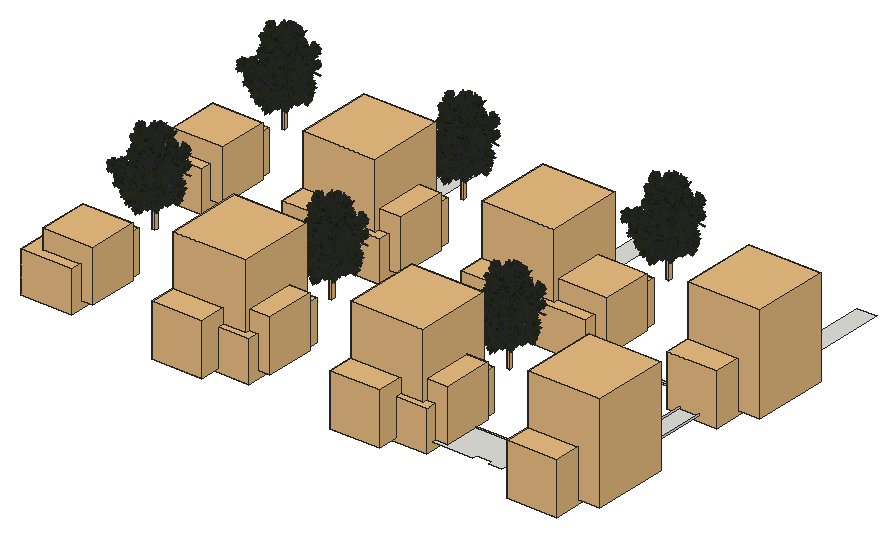
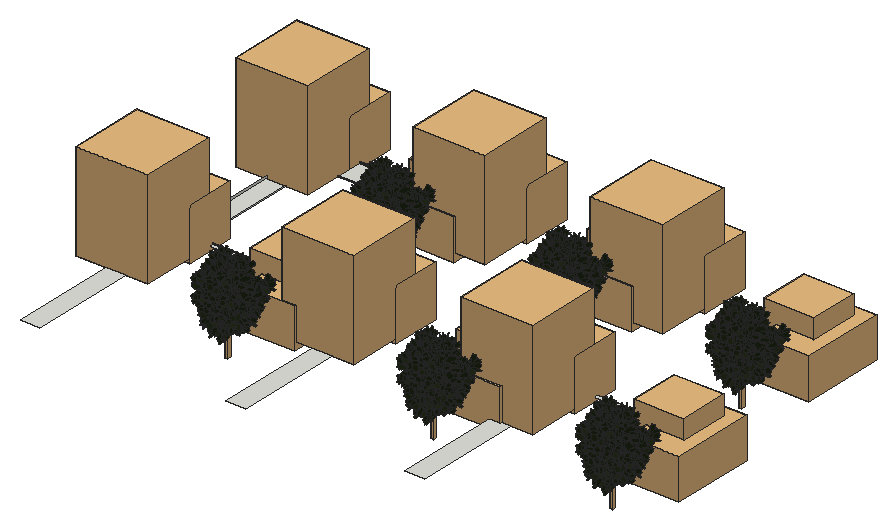
# SketchUp Ruby script. Lengths in inches.
U = 1.inch
M = Sketchup.active_model
def pt(a) = Geom::Point3d.new(a.map { |v| v * U })
def face(e, loops, mat)
  f = e.add_face(loops[0].map { |a| pt(a) })
  loops[1..].each { |l| e.add_face(l.map { |a| pt(a) }).erase! }
  f.material = f.back_material = mat if mat
  f
end
# faces: each face lists its corners as indices into pts; further lists are holes
def faces(e, pts, list, mat = nil) = list.each { |f| face(e, (f[0].is_a?(Array) ? f : [f]).map { |l| l.map { |i| pts[i] } }, mat) }
# xy, xz, yz: faces in a plane at the given z, y or x. An outline is a flat list of corners, or four numbers for a rectangle; further outlines are holes
def ring(l) = l.size == 4 ? [[l[0], l[1]], [l[2], l[1]], [l[2], l[3]], [l[0], l[3]]] : l.each_slice(2).to_a
def flat(e, list, mat, &to3) = list.each { |f| face(e, (f[0].is_a?(Array) ? f : [f]).map { |l| ring(l).map { |u, v| to3.(u, v) } }, mat) }
def xy(e, z, list, mat = nil) = flat(e, list, mat) { |x, y| [x, y, z] }
def xz(e, y, list, mat = nil) = flat(e, list, mat) { |x, z| [x, y, z] }
def yz(e, x, list, mat = nil) = flat(e, list, mat) { |y, z| [x, y, z] }
def lines(e, pts, list) = list.each { |a, b| e.add_line(pt(pts[a]), pt(pts[b])) }
# prism: a flat outline (further loops are holes) pulled along v
def prism(e, loops, v, mat = nil)
  f = face(e, loops, mat); d = Geom::Vector3d.new(v.map { |x| x * U })
  f.pushpull(f.normal.samedirection?(d) ? d.length : -d.length)
end
def box(e, o, s, mat = nil) = prism(e, [[o, [o[0] + s[0], o[1], o[2]], [o[0] + s[0], o[1] + s[1], o[2]], [o[0], o[1] + s[1], o[2]]]], [0, 0, s[2]], mat)
def at(x, y, z, deg = 0) = Geom::Transformation.translation(pt([x, y, z])) * Geom::Transformation.rotation(ORIGIN, Z_AXIS, deg.degrees)
def axes(o, x, y, z) = Geom::Transformation.new([*x, 0, *y, 0, *z, 0, *pt(o).to_a, 1])
def part(name) = M.definitions.add(name)
# library, detail: a bought-in or finely detailed component or shape, given as its bounding box
def library(name, o, s) = part(name).tap { |d| box(d.entities, o, s) }
def detail(e, o, s) = box(e.add_group.entities, o, s)
def put(e, d, t, mat = nil) = e.add_instance(d, t).tap { |i| i.material = mat if mat }
def group(e, t, mat = nil) = e.add_group.tap { |g| g.transformation = t; g.material = mat if mat }.entities
root = M.entities
M.materials.add("Green ash – green texture").color = [33, 41, 22]
M.materials.add("[Color_005]").color = [114, 114, 114]
M.materials.add("[Color_D09]").color = [86, 59, 49]
M.materials.add("[Pavers with Grass Herringbone]").color = [197, 201, 190]
c1 = part("Component\#13")
xz(c1.entities,0,[[2.54,0,9.87,0.64,10.99,2.07,11.4,3.42,15.13,2.28,14.48,4.31,16.14,5.21,16.14,6.08,19.81,7.28,19.6,9.67,17.45,11.49,17.45,12.16,18.82,14.37,17.48,14.37,14.41,13.66,14.41,15.23,12.5625,17.49,9.84,15.21,8.9,13.85,7.74,13.625,7.35,12.68,6.87,13.02,6.35,12.27,5.92,10.47,4.2,7.42,2.84,6.89,0,2.38,0.07,1.59,2.8125,4.94,3.37,3.59,2.54,3.37,2.12,2.22]],"Green ash – green texture")
c2 = part("Component\#14")
xz(c2.entities,0,[[1.1,0,1.61,0,2.73,1.11,4.34,2.72,5.21,6.36,5.85,7.16,6.35,6.9375,6.85,8.05,8.03,8.05,8.625,9.25,10.11,11.7,9.56,13.83,9.56,15.84,7.83,15.84,6.03,14.37,5.31,16.54,4.4375,17.39,1.45,14.31,0,9.15,1.4,5.18,3.01,6.08,1.98,1.39]],"Green ash – green texture")
c3 = part("Component\#16")
put(c3.entities,c1,axes([0,7.77,0],[1,0,0],[0,0.89571,0.44464],[0,-0.44464,0.89571]))
put(c3.entities,c2,axes([2.15,6.37,5.26],[0.57629,-0.80824,0.12095],[0.79263,0.51673,-0.3236],[0.19905,0.28236,0.93843]))
c4 = part("Component\#7")
put(c4.entities,c3,axes([-4.97,-3.22,4.05],[0.69883,-0.69034,0.18725],[0.53248,0.3273,-0.7806],[0.47759,0.64522,0.59632]))
c5 = part("Component\#8")
put(c5.entities,c4,axes([0,5.2,2.2],[1,0,0],[0,0.90259,0.43051],[0,-0.43051,0.90259]))
c6 = part("leaf group 2")
put(c6.entities,c5,axes([-11.99,4.41,-4.35],[2.22014,-0.82385,1.14017],[1.36501,1.77637,-1.37441],[-0.33979,1.75315,1.92841]))
c7 = part("Component\#10")
put(c7.entities,c6,axes([-5.27,11.65,1.68],[-0.48323,0.10636,-0.43072],[-0.11515,-0.64511,-0.03012],[-0.42845,0.05342,0.49388]))
c8 = part("Component\#9")
xz(c8.entities,0,[[0.64,0,0,0.1875,4.21,2.81,8.59,4.11,12.8,4.11,19.57,2.81,12.8,3.73,8.59,3.73,4.21,2.3125]],"[Color_D09]")
c9 = part("Leafy twig")
put(c9.entities,c7,axes([23.53,12.57,24.85],[0.06536,-0.90475,-0.42089],[0.61791,-0.2945,0.72901],[-0.78353,-0.30772,0.53981]))
put(c9.entities,c7,axes([22.7,12.25,24.83],[-0.47146,-0.89493,0.11311],[0.80135,-0.48549,-0.35888],[0.36776,-0.0521,0.90651]))
put(c9.entities,c7,axes([24.25,0.65,20.83],[0.8253,-0.50372,0.24924],[0.23848,0.71461,0.65749],[-0.51157,-0.48438,0.71194]))
put(c9.entities,c7,axes([23.54,-2.45,18.63],[0.04689,-0.92492,0.3511],[0.72122,-0.28285,-0.64421],[0.71641,0.2674,0.65188]))
put(c9.entities,c7,axes([22.39,16.15,27.04],[-0.5311,-0.82173,0.2419],[0.41574,0.01583,0.89559],[-0.77461,0.50499,0.40813]))
put(c9.entities,c8,axes([22.76,-5.09,13.48],[0,1.66539,0.44624],[-1.72414,0,0],[0,-0.44624,1.66539]))
c10 = part("Component\#12")
p = [[0,0,0.13],[0.41,0.77,0],[4.07,2.79,10.125],[3.73,2.15,10.23],[7.66,4.77,23.875],[7.4,4.27,23.96],
  [8.6875,5.26,35.99],[8.5,4.91,36.05],[8.32,4.9375,46.95],[8.21,4.74,46.98]]
faces(c10.entities,p,[[0,1,2,3],[3,2,4,5],[4,6,7,5],[6,8,9,7]],"[Color_005]")
c11 = part("Leafy twig \#1")
put(c11.entities,c10,axes([3.13,0.17,-0.45],[3.38032,6.88592,0.52481],[-5.85488,3.97559,0.303],[0,-1.35912,3.54524]))
put(c11.entities,c7,axes([0.37,31.375,148.94],[0.47772,0.64064,-1.51139],[2.85768,-0.62659,0.20284],[-0.43926,-3.3797,-0.3241]))
c12 = part("Leafy branch \#1")
put(c12.entities,c9,axes([28.11,72.66,46.26],[0.77413,-0.41274,-0.47998],[0.6311,0.56229,0.53435],[0.04934,-0.71657,0.69577]))
put(c12.entities,c9,axes([31.25,3.94,9.17],[0.73236,0.67893,0.05208],[-0.46223,0.55185,-0.69413],[-0.5,0.48428,0.71797]))
put(c12.entities,c9,axes([20.16,84.84,57.95],[0.96628,0.19619,0.16678],[-0.2575,0.73909,0.62245],[-0.00115,-0.6444,0.76469]))
put(c12.entities,c9,axes([30.13,29.18,11.93],[0.86603,0.2796,0.41452],[0,0.82904,-0.55919],[-0.5,0.48428,0.71797]))
put(c12.entities,c9,axes([47.67,28.63,-3.7],[0.1205,-0.71255,0.69119],[0.96646,0.24327,0.08231],[-0.2268,0.65809,0.71797]))
put(c12.entities,c9,axes([48.76,50.64,76.31],[-0.6716,0.46861,-0.57389],[0.01402,0.78248,0.62252],[0.74078,0.41004,-0.53209]))
put(c12.entities,c11,axes([42.34,0,10.34],[0.39368,0,0],[0,0.22544,-0.24092],[0,0.54032,0.50562]))
put(c12.entities,c9,axes([64.51,80.82,101.08],[-0.99604,0.06562,-0.06004],[-0.0106,0.58266,0.81265],[0.08831,0.81006,-0.57966]))
c13 = library("Component\#18",[-6.35,9.4375,-76.57],[12.56,13.68,315.77])
c14 = part("Leafy branch \#3")
put(c14.entities,c9,axes([-3.64,36.17,23.18],[0.95801,0.10249,0.26779],[-0.28581,0.41631,0.86313],[-0.02302,-0.90343,0.42812]))
put(c14.entities,c9,axes([13.16,55.79,39.92],[0.70711,-0.61725,0.34497],[0,0.48786,0.87292],[-0.70711,-0.61725,0.34497]))
put(c14.entities,c11,axes([18.8125,5.17,0.46],[0.25503,0,0],[0,0.20007,-0.0752],[0,0.16866,0.44872]))
put(c14.entities,c9,axes([23.62,-10.17,21.5],[-0.56253,0.81775,0.12181],[0.38738,0.13053,0.91263],[0.73041,0.56057,-0.39021]))
put(c14.entities,c9,axes([45.18,27.18,68.96],[-0.96593,-0.22593,0.12627],[0.12295,0.02876,0.992],[-0.22775,0.97372,0]))
c15 = part("Component\#19")
put(c15.entities,c11,axes([21.47,3.93,0.22],[0.25503,0,0],[0,0.21068,-0.03601],[0,0.08077,0.47252]))
put(c15.entities,c9,axes([-4.05,13.6875,55.34],[0.70711,0.70373,-0.069],[0,0.09758,0.99523],[0.70711,-0.70373,0.069]))
put(c15.entities,c9,axes([6.52,33.54,18.07],[0.92587,-0.37604,0.03687],[0,0.09758,0.99523],[-0.37784,-0.92145,0.09035]))
c16 = part("Leafy branch \#2")
put(c16.entities,c9,axes([26.17,74.02,40.56],[0.25882,-0.64004,0.72344],[0,0.74896,0.66262],[-0.96593,-0.1715,0.19384]))
put(c16.entities,c9,axes([6.38,24.03,55.81],[-0.04786,0.8645,-0.50035],[0.15558,0.50126,0.85119],[0.98666,-0.03711,-0.15849]))
put(c16.entities,c11,axes([17.68,0,1.01],[0.32282,0,0],[0,0.21407,-0.16545],[0,0.37107,0.48011]))
put(c16.entities,c9,axes([-9.1875,31.15,28.07],[0.82314,0.37626,-0.42529],[0,0.74896,0.66262],[0.56784,-0.54543,0.61649]))
put(c16.entities,c9,axes([0.54,-12.07,9.94],[0.19622,0.90478,-0.37799],[-0.67396,0.40444,0.61823],[0.71224,0.13344,0.68914]))
put(c16.entities,c9,axes([7.34,9.15,39.57],[0.05153,0.73872,-0.67204],[0.38679,0.60565,0.6954],[0.92072,-0.29578,-0.25452]))
put(c16.entities,c9,axes([36.2,51.23,15.73],[-0.18626,-0.35374,0.91661],[-0.31641,0.90483,0.2849],[-0.93016,-0.23696,-0.28046]))
c17 = part("Tree")
put(c17.entities,c12,axes([-22.29,52.36,216.76],[0.38964,-1.07313,-0.10036],[1.06809,0.37236,0.19631],[-0.13881,-0.14712,1.22884]))
put(c17.entities,c12,axes([59.83,6.78,230.57],[-1.28826,-0.23008,-0.3647],[0.05148,-1.22938,0.51215],[-0.34663,0.55136,1.25774]))
put(c17.entities,c13,axes([-2.16,-18.04,104.22],[1.30157,0,0],[0,1.30157,0],[0,0,1.36111]))
put(c17.entities,c12,axes([-55.8,4.2,115.32],[1.30157,0,0],[0,1.29536,0.19359],[0,-0.26855,1.38538]))
put(c17.entities,c12,axes([5.36,-52.22,156.04],[-0.23532,1.19719,-0.71362],[-1.32974,0,0.39335],[0.40758,0.6912,1.23603]))
put(c17.entities,c14,axes([-20.09,22.57,317.7],[0,-1.33697,0],[1.33697,0,0],[0,0,1.4573]))
put(c17.entities,c12,axes([44.2,-31.84,172.82],[-1.11894,0.85085,0],[-0.85085,-1.11894,0],[0,0,1.53221]))
put(c17.entities,c12,axes([-10.2,63.7,119.93],[0.28716,-1.46366,0],[1.41378,0.27737,0.38604],[-0.41292,-0.08101,1.5704]))
put(c17.entities,c12,axes([-29.03,-40.72,232.79],[0.5211,0.98898,-0.38718],[-1.02974,0.58664,0.11255],[0.35577,0.28216,1.19957]))
put(c17.entities,c12,axes([44.92,21.7,135.38],[-1.05627,-0.44294,0],[0.44294,-1.05627,0],[0,0,1.24847]))
put(c17.entities,c14,axes([-32.94,-0.59,304.82],[1.2814,-0.22825,0],[0.22825,1.2814,0],[0,0,1.41871]))
put(c17.entities,c14,axes([0.6,-31.29,315.98],[0.13082,1.33422,0],[-1.33422,0.13082,0],[0,0,1.46127]))
put(c17.entities,c14,axes([21.3,1.66,315.16],[-1.25722,0.32198,-0.09905],[-0.32539,-1.26867,0.00612],[-0.08719,0.09194,1.40547]))
put(c17.entities,c15,axes([-19,30.84,372.72],[0.65078,-1.12719,0],[1.12719,0.65078,0],[0,0,1.41871]))
put(c17.entities,c15,axes([14.39,-16.125,357],[-0.73695,1.06095,0.15933],[-1.03698,-0.75397,0.2242],[0.29981,0,1.38667]))
put(c17.entities,c16,axes([-5.9,-20.03,270.39],[0,1.47598,0],[-1.4157,0,0.41751],[0.45509,0,1.54311]))
put(c17.entities,c16,axes([-18.4375,22.18,263.88],[0.84243,-1.42226,-0.32685],[1.40385,0.7063,0.64743],[-0.37678,-0.54841,1.68147]))
put(c17.entities,c16,axes([-29.32,4.9,283.41],[1.35363,0,0],[0,1.33841,0.20242],[0,-0.22063,1.45887]))
put(c17.entities,c16,axes([17.31,11.65,257.52],[-1.14969,-0.5642,-0.25322],[0.46017,-1.12719,0.50159],[-0.40066,0.32434,1.3027]))
put(c17.entities,c16,axes([16.3,15.3125,240.45],[-0.98541,-0.85203,0.68095],[1.00747,-1.01506,0.22317],[0.31818,0.5753,1.40228]))
put(c17.entities,c12,axes([-46.75,22.93,206.12],[1.08363,-0.37101,0],[0.37101,1.08363,0],[0,0,1.24847]))
put(c17.entities,c12,axes([41.1,-35.18,99.125],[-1.05556,0.85173,0.25344],[-0.84493,-1.04965,0.12953],[0.39153,-0.09409,1.38106]))
c18 = library("VEGETAÇÃO+TROPICAL+EM+VASOS",[-14.15,-83.94,15.25],[179.21,109.09,86.78])
c19 = library("Plant+++Pot",[-21.48,-119.36,-205.6875],[86.44,86.43,89.41])
c20 = library("Plant",[0,0,0],[12.59,12.59,14.16])
c21 = library("ganyedes's+yellow&green+tree",[-30.91,-35.46,0],[63.51,67.02,85.79])
xy(root,-12.3125,[[2364.02,147.25,2435.71,305.58],[2140.42,162.33,2140.42,178.0625,2083.4,178.0625,2083.4,162.52,1785.21,162.52,1785.21,305.58,2364.02,305.58,2364.02,203.875,2347.875,203.875,2347.875,204.875,2347.125,204.875,2347.125,203.875,2343.875,203.875,2343.875,204.875,2343.125,204.875,2343.125,203.875,2339.875,203.875,2339.875,204.875,2339.125,204.875,2339.125,203.875,2335.875,203.875,2335.875,204.875,2335.125,204.875,2335.125,203.875,2331.875,203.875,2331.875,204.875,2331.125,204.875,2331.125,203.875,2327.875,203.875,2327.875,204.875,2327.125,204.875,2327.125,203.875,2323.875,203.875,2323.875,204.875,2323.125,204.875,2323.125,203.875,2319.875,203.875,2319.875,204.875,2319.125,204.875,2319.125,203.875,2315.875,203.875,2315.875,204.875,2315.125,204.875,2315.125,203.875,2311.875,203.875,2311.875,204.875,2311.125,204.875,2311.125,203.875,2307.875,203.875,2307.875,204.875,2307.125,204.875,2307.125,203.875,2303.875,203.875,2303.875,204.875,2303.125,204.875,2303.125,203.875,2299.875,203.875,2299.875,204.875,2299.125,204.875,2299.125,203.875,2295.875,203.875,2295.875,204.875,2295.125,204.875,2295.125,203.875,2291.875,203.875,2291.875,204.875,2291.125,204.875,2291.125,203.875,2287.875,203.875,2287.875,204.875,2287.125,204.875,2287.125,203.875,2283.875,203.875,2283.875,204.875,2283.125,204.875,2283.125,203.875,2279.875,203.875,2279.875,204.875,2279.125,204.875,2279.125,203.875,2275.875,203.875,2275.875,204.875,2275.125,204.875,2275.125,203.875,2271.875,203.875,2271.875,204.875,2271.125,204.875,2271.125,203.875,2267.875,203.875,2267.875,204.875,2267.125,204.875,2267.125,203.875,2263.875,203.875,2263.875,204.875,2263.125,204.875,2263.125,203.875,2259.875,203.875,2259.875,204.875,2259.125,204.875,2259.125,203.875,2255.875,203.875,2255.875,204.875,2255.125,204.875,2255.125,203.875,2251.875,203.875,2251.875,204.875,2251.125,204.875,2251.125,203.875,2247.875,203.875,2247.875,204.875,2247.125,204.875,2247.125,203.875,2243.875,203.875,2243.875,204.875,2243.125,204.875,2243.125,203.875,2239.875,203.875,2239.875,204.875,2239.125,204.875,2239.125,203.875,2235.875,203.875,2235.875,204.875,2235.125,204.875,2235.125,203.875,2231.875,203.875,2231.875,204.875,2231.125,204.875,2231.125,203.875,2227.875,203.875,2227.875,204.875,2227.125,204.875,2227.125,203.875,2223.875,203.875,2223.875,204.875,2223.125,204.875,2223.125,203.875,2219.875,203.875,2219.875,204.875,2219.125,204.875,2219.125,203.875,2215.875,203.875,2215.875,204.875,2215.125,204.875,2215.125,203.875,2211.875,203.875,2211.875,204.875,2211.125,204.875,2211.125,203.875,2207.875,203.875,2207.875,204.875,2207.125,204.875,2207.125,203.875,2203.875,203.875,2203.875,204.875,2203.125,204.875,2203.125,203.875,2199.875,203.875,2199.875,204.875,2199.125,204.875,2199.125,203.875,2195.875,203.875,2195.875,204.875,2195.125,204.875,2195.125,203.875,2191.875,203.875,2191.875,204.875,2191.125,204.875,2191.125,203.875,2189.5,203.875,2189.5,162.33],[2364.02,305.58,2435.71,838.14],[811.8125,838.14,986.33,853.22],[986.33,838.14,1058.02,996.48],
  [1641.83,838.14,1713.52,996.48],[2221.9375,838.14,2396.46,853.22],[2396.46,838.14,2468.15,996.48],[986.33,996.48,1058.02,1529.04],[1641.83,996.48,1713.52,1529.04],
  [2396.46,996.48,2468.15,1529.04]])
xz(root,147.25,[[2364.02,-12.3125,2435.71,-4.67]])
xz(root,204.875,[[2191.125,-12.3125,2191.875,-8],[2195.125,-12.3125,2195.875,-8],[2215.125,-12.3125,2215.875,-8],[2223.125,-12.3125,2223.875,-8],[2227.125,-12.3125,2227.875,-8],
  [2231.125,-12.3125,2231.875,-8],[2235.125,-12.3125,2235.875,-8],[2239.125,-12.3125,2239.875,-8],[2243.125,-12.3125,2243.875,-8],[2247.125,-12.3125,2247.875,-8],
  [2251.125,-12.3125,2251.875,-8],[2255.125,-12.3125,2255.875,-8],[2259.125,-12.3125,2259.875,-8],[2263.125,-12.3125,2263.875,-8],[2267.125,-12.3125,2267.875,-8],
  [2271.125,-12.3125,2271.875,-8],[2275.125,-12.3125,2275.875,-8],[2279.125,-12.3125,2279.875,-8],[2283.125,-12.3125,2283.875,-8],[2287.125,-12.3125,2287.875,-8],
  [2291.125,-12.3125,2291.875,-8],[2295.125,-12.3125,2295.875,-8],[2299.125,-12.3125,2299.875,-8],[2303.125,-12.3125,2303.875,-8],[2307.125,-12.3125,2307.875,-8],
  [2311.125,-12.3125,2311.875,-8],[2315.125,-12.3125,2315.875,-8],[2319.125,-12.3125,2319.875,-8],[2323.125,-12.3125,2323.875,-8],[2327.125,-12.3125,2327.875,-8],
  [2331.125,-12.3125,2331.875,-8],[2335.125,-12.3125,2335.875,-8],[2339.125,-12.3125,2339.875,-8],[2343.125,-12.3125,2343.875,-8],[2347.125,-12.3125,2347.875,-8]])
xz(root,305.58,[[1785.21,-12.3125,2364.02,-8],[2364.02,-12.3125,2435.71,-4.67]])
xz(root,838.14,[[953.9,-12.3125,986.33,-8],[986.33,-12.3125,1025.58,-8],[1983.13,-12.3125,2364.02,-8],[2364.02,-12.3125,2396.46,-8],[2396.46,-12.3125,2435.71,-8],
  [2435.71,-12.3125,2468.15,-8]])
xz(root,996.48,[[986.33,-12.3125,1058.02,-4.67],[1641.83,-12.3125,1713.52,-4.67],[2396.46,-12.3125,2468.15,-4.67]])
yz(root,2191.125,[[203.875,-12.3125,204.875,-8]])
yz(root,2191.875,[[203.875,-12.3125,204.875,-8]])
yz(root,2195.125,[[203.875,-12.3125,204.875,-8]])
yz(root,2207.875,[[203.875,-12.3125,204.875,-8]])
yz(root,2211.125,[[203.875,-12.3125,204.875,-8]])
yz(root,2223.125,[[203.875,-12.3125,204.875,-8]])
yz(root,2223.875,[[203.875,-12.3125,204.875,-8]])
yz(root,2227.125,[[203.875,-12.3125,204.875,-8]])
yz(root,2227.875,[[203.875,-12.3125,204.875,-8]])
yz(root,2231.125,[[203.875,-12.3125,204.875,-8]])
yz(root,2231.875,[[203.875,-12.3125,204.875,-8]])
yz(root,2235.125,[[203.875,-12.3125,204.875,-8]])
yz(root,2235.875,[[203.875,-12.3125,204.875,-8]])
yz(root,2239.125,[[203.875,-12.3125,204.875,-8]])
yz(root,2239.875,[[203.875,-12.3125,204.875,-8]])
yz(root,2243.125,[[203.875,-12.3125,204.875,-8]])
yz(root,2243.875,[[203.875,-12.3125,204.875,-8]])
yz(root,2247.125,[[203.875,-12.3125,204.875,-8]])
yz(root,2247.875,[[203.875,-12.3125,204.875,-8]])
yz(root,2251.125,[[203.875,-12.3125,204.875,-8]])
yz(root,2251.875,[[203.875,-12.3125,204.875,-8]])
yz(root,2255.125,[[203.875,-12.3125,204.875,-8]])
yz(root,2255.875,[[203.875,-12.3125,204.875,-8]])
yz(root,2259.125,[[203.875,-12.3125,204.875,-8]])
yz(root,2259.875,[[203.875,-12.3125,204.875,-8]])
yz(root,2263.125,[[203.875,-12.3125,204.875,-8]])
yz(root,2263.875,[[203.875,-12.3125,204.875,-8]])
yz(root,2267.125,[[203.875,-12.3125,204.875,-8]])
yz(root,2267.875,[[203.875,-12.3125,204.875,-8]])
yz(root,2271.125,[[203.875,-12.3125,204.875,-8]])
yz(root,2271.875,[[203.875,-12.3125,204.875,-8]])
yz(root,2275.125,[[203.875,-12.3125,204.875,-8]])
yz(root,2275.875,[[203.875,-12.3125,204.875,-8]])
yz(root,2279.125,[[203.875,-12.3125,204.875,-8]])
yz(root,2279.875,[[203.875,-12.3125,204.875,-8]])
yz(root,2283.125,[[203.875,-12.3125,204.875,-8]])
yz(root,2283.875,[[203.875,-12.3125,204.875,-8]])
yz(root,2287.125,[[203.875,-12.3125,204.875,-8]])
yz(root,2287.875,[[203.875,-12.3125,204.875,-8]])
yz(root,2291.125,[[203.875,-12.3125,204.875,-8]])
yz(root,2291.875,[[203.875,-12.3125,204.875,-8]])
yz(root,2295.125,[[203.875,-12.3125,204.875,-8]])
yz(root,2295.875,[[203.875,-12.3125,204.875,-8]])
yz(root,2299.125,[[203.875,-12.3125,204.875,-8]])
yz(root,2299.875,[[203.875,-12.3125,204.875,-8]])
yz(root,2303.125,[[203.875,-12.3125,204.875,-8]])
yz(root,2303.875,[[203.875,-12.3125,204.875,-8]])
yz(root,2307.125,[[203.875,-12.3125,204.875,-8]])
yz(root,2307.875,[[203.875,-12.3125,204.875,-8]])
yz(root,2311.125,[[203.875,-12.3125,204.875,-8]])
yz(root,2311.875,[[203.875,-12.3125,204.875,-8]])
yz(root,2315.125,[[203.875,-12.3125,204.875,-8]])
yz(root,2315.875,[[203.875,-12.3125,204.875,-8]])
yz(root,2319.125,[[203.875,-12.3125,204.875,-8]])
yz(root,2319.875,[[203.875,-12.3125,204.875,-8]])
yz(root,2323.125,[[203.875,-12.3125,204.875,-8]])
yz(root,2323.875,[[203.875,-12.3125,204.875,-8]])
yz(root,2327.125,[[203.875,-12.3125,204.875,-8]])
yz(root,2327.875,[[203.875,-12.3125,204.875,-8]])
yz(root,2331.125,[[203.875,-12.3125,204.875,-8]])
yz(root,2331.875,[[203.875,-12.3125,204.875,-8]])
yz(root,2335.125,[[203.875,-12.3125,204.875,-8]])
yz(root,2335.875,[[203.875,-12.3125,204.875,-8]])
yz(root,2339.125,[[203.875,-12.3125,204.875,-8]])
yz(root,2339.875,[[203.875,-12.3125,204.875,-8]])
yz(root,2343.125,[[203.875,-12.3125,204.875,-8]])
yz(root,2343.875,[[203.875,-12.3125,204.875,-8]])
yz(root,2347.125,[[203.875,-12.3125,204.875,-8]])
yz(root,2347.875,[[203.875,-12.3125,204.875,-8]])
yz(root,2364.02,[[203.875,-12.3125,305.58,-8],[305.58,-12.3125,838.14,-8]])
yz(root,2435.71,[[147.25,-12.3125,305.58,-4.67],[305.58,-12.3125,838.14,-4.67]])
put(root,c17,axes([1838.53,634.3125,-12.15],[0.68,0,0],[0,0.68,0],[0,0,0.68]))
put(root,c17,axes([1188.03,634.3125,-12.15],[0.68,0,0],[0,0.68,0],[0,0,0.68]))
put(root,c17,axes([1116.34,1325.21,-12.15],[0.68,0,0],[0,0.68,0],[0,0,0.68]))
put(root,c17,axes([1870.97,1325.21,-12.15],[0.68,0,0],[0,0.68,0],[0,0,0.68]))
put(root,c17,axes([460.84,1325.21,-12.15],[0.68,0,0],[0,0.68,0],[0,0,0.68]))
put(root,c17,axes([537.53,634.3125,-12.15],[0.68,0,0],[0,0.68,0],[0,0,0.68]))
put(root,c18,axes([1888.3,423.09,-68.95],[0,-1.727,0],[1.727,0,0],[0,0,1.727]))
put(root,c18,axes([1237.8,423.09,-68.95],[0,-1.727,0],[1.727,0,0],[0,0,1.727]))
put(root,c18,axes([1166.11,1113.98,-68.95],[0,-1.727,0],[1.727,0,0],[0,0,1.727]))
put(root,c18,axes([1920.73,1113.98,-68.95],[0,-1.727,0],[1.727,0,0],[0,0,1.727]))
put(root,c18,axes([510.61,1113.98,-68.95],[0,-1.727,0],[1.727,0,0],[0,0,1.727]))
put(root,c18,axes([587.3,423.09,-68.95],[0,-1.727,0],[1.727,0,0],[0,0,1.727]))
put(root,c19,axes([2330.29,318.71,404.95],[2.12,0,0],[0,2.12,0],[0,0,2.12]))
put(root,c19,axes([1679.79,318.71,404.95],[2.12,0,0],[0,2.12,0],[0,0,2.12]))
put(root,c19,axes([1608.1,1009.61,404.95],[2.12,0,0],[0,2.12,0],[0,0,2.12]))
put(root,c19,axes([2362.73,1009.61,404.95],[2.12,0,0],[0,2.12,0],[0,0,2.12]))
put(root,c19,axes([952.6,1009.61,404.95],[2.12,0,0],[0,2.12,0],[0,0,2.12]))
put(root,c19,axes([1029.29,318.71,404.95],[2.12,0,0],[0,2.12,0],[0,0,2.12]))
put(root,c20,axes([2366.39,272.32,-19.08],[2.21,0,0],[0,2.21,0],[0,0,2.21]))
put(root,c20,axes([1715.89,272.32,-19.08],[2.21,0,0],[0,2.21,0],[0,0,2.21]),"[Pavers with Grass Herringbone]")
put(root,c20,axes([1644.2,963.21,-19.08],[2.21,0,0],[0,2.21,0],[0,0,2.21]))
put(root,c20,axes([2398.83,963.21,-19.08],[2.21,0,0],[0,2.21,0],[0,0,2.21]))
put(root,c20,axes([988.7,963.21,-19.08],[2.21,0,0],[0,2.21,0],[0,0,2.21]))
put(root,c20,axes([1065.39,272.32,-19.08],[2.21,0,0],[0,2.21,0],[0,0,2.21]))
put(root,c21,axes([2413.66,309.92,-13.42],[4.17,0,0],[0,4.17,0],[0,0,4.17]))
put(root,c21,axes([1763.16,309.92,-13.42],[4.17,0,0],[0,4.17,0],[0,0,4.17]))
put(root,c21,axes([1691.47,1000.8125,-13.42],[4.17,0,0],[0,4.17,0],[0,0,4.17]))
put(root,c21,axes([2446.1,1000.8125,-13.42],[4.17,0,0],[0,4.17,0],[0,0,4.17]))
put(root,c21,axes([1035.97,1000.8125,-13.42],[4.17,0,0],[0,4.17,0],[0,0,4.17]))
put(root,c21,axes([1112.66,309.92,-13.42],[4.17,0,0],[0,4.17,0],[0,0,4.17]))
put(root,c19,axes([1838.875,430.97,423.1],[2.12,0,0],[0,2.12,0],[0,0,2.12]))
put(root,c19,axes([1188.375,430.97,423.1],[2.12,0,0],[0,2.12,0],[0,0,2.12]))
put(root,c19,axes([1116.6875,1121.86,423.1],[2.12,0,0],[0,2.12,0],[0,0,2.12]))
put(root,c19,axes([1871.3125,1121.86,423.1],[2.12,0,0],[0,2.12,0],[0,0,2.12]))
put(root,c19,axes([461.1875,1121.86,423.1],[2.12,0,0],[0,2.12,0],[0,0,2.12]))
put(root,c19,axes([537.875,430.97,423.1],[2.12,0,0],[0,2.12,0],[0,0,2.12]))
